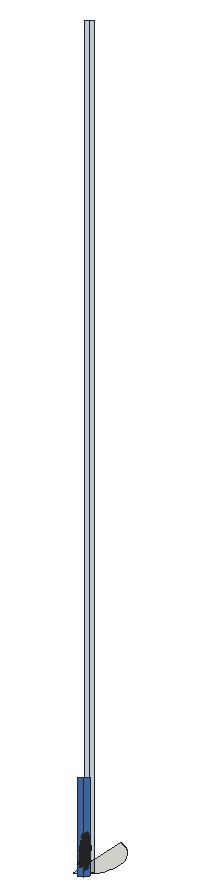
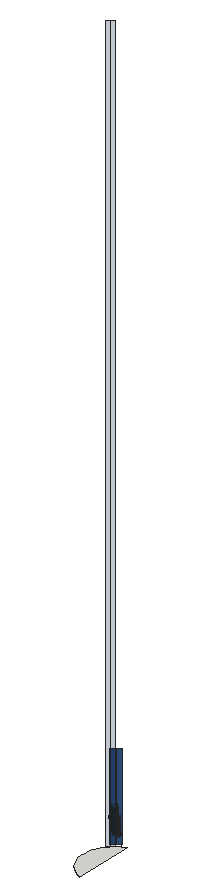
# SketchUp Ruby script. Lengths in inches.
U = 1.inch
M = Sketchup.active_model
def pt(a) = Geom::Point3d.new(a.map { |v| v * U })
def face(e, loops, mat)
  f = e.add_face(loops[0].map { |a| pt(a) })
  loops[1..].each { |l| e.add_face(l.map { |a| pt(a) }).erase! }
  f.material = f.back_material = mat if mat
  f
end
# faces: each face lists its corners as indices into pts; further lists are holes
def faces(e, pts, list, mat = nil) = list.each { |f| face(e, (f[0].is_a?(Array) ? f : [f]).map { |l| l.map { |i| pts[i] } }, mat) }
# xy, xz, yz: faces in a plane at the given z, y or x. An outline is a flat list of corners, or four numbers for a rectangle; further outlines are holes
def ring(l) = l.size == 4 ? [[l[0], l[1]], [l[2], l[1]], [l[2], l[3]], [l[0], l[3]]] : l.each_slice(2).to_a
def flat(e, list, mat, &to3) = list.each { |f| face(e, (f[0].is_a?(Array) ? f : [f]).map { |l| ring(l).map { |u, v| to3.(u, v) } }, mat) }
def xy(e, z, list, mat = nil) = flat(e, list, mat) { |x, y| [x, y, z] }
def xz(e, y, list, mat = nil) = flat(e, list, mat) { |x, z| [x, y, z] }
def yz(e, x, list, mat = nil) = flat(e, list, mat) { |y, z| [x, y, z] }
def lines(e, pts, list) = list.each { |a, b| e.add_line(pt(pts[a]), pt(pts[b])) }
# prism: a flat outline (further loops are holes) pulled along v
def prism(e, loops, v, mat = nil)
  f = face(e, loops, mat); d = Geom::Vector3d.new(v.map { |x| x * U })
  f.pushpull(f.normal.samedirection?(d) ? d.length : -d.length)
end
def box(e, o, s, mat = nil) = prism(e, [[o, [o[0] + s[0], o[1], o[2]], [o[0] + s[0], o[1] + s[1], o[2]], [o[0], o[1] + s[1], o[2]]]], [0, 0, s[2]], mat)
def at(x, y, z, deg = 0) = Geom::Transformation.translation(pt([x, y, z])) * Geom::Transformation.rotation(ORIGIN, Z_AXIS, deg.degrees)
def axes(o, x, y, z) = Geom::Transformation.new([*x, 0, *y, 0, *z, 0, *pt(o).to_a, 1])
def part(name) = M.definitions.add(name)
# library, detail: a bought-in or finely detailed component or shape, given as its bounding box
def library(name, o, s) = part(name).tap { |d| box(d.entities, o, s) }
def detail(e, o, s) = box(e.add_group.entities, o, s)
def put(e, d, t, mat = nil) = e.add_instance(d, t).tap { |i| i.material = mat if mat }
def group(e, t, mat = nil) = e.add_group.tap { |g| g.transformation = t; g.material = mat if mat }.entities
root = M.entities
M.materials.add("Glass_Basic_1").color = [0, 47, 91]
M.materials["Glass_Basic_1"].alpha = 0.25
M.materials.add("Glass_Mirror_01").color = [71, 118, 185]
M.materials.add("LightPink_Translucent").color = [144, 107, 117]
M.materials["LightPink_Translucent"].alpha = 0.75
c1 = part("blade")
p = [[2.15,0.21,22],[0,0.17,0],[0.09,0.45,0],[2.18,0.31,22],[2.29,0.31,22],[0.38,0.45,0],
  [2.48,0.24,33],[2.49,0.24,33],[2.48,0.22,33]]
faces(c1.entities,p,[[0,1,2,3],[4,5,2,3],[6,3,4,7],[8,0,3,6]])
c2 = part("seeds")
p = [[0.3,-0.1,1.38],[-0.01,-0.03,1.59],[-0.01,-0.03,0.03],[0.14,-0.07,-0.07],[0.29,-0.03,3],[0.15,0.01,3.11]]
faces(c2.entities,p,[[0,1,2,3],[1,0,4,5]],"LightPink_Translucent")
c3 = part("blade with seeds")
put(c3.entities,c1,at(0,0,0))
put(c3.entities,c2,axes([2.4,0.25,30.99],[1.5799,-0.05474,1.17369],[-0.12525,1.92788,0.29478],[-0.07173,-0.02425,1.56792]))
xy(root,-24,[[330.57,22.73,330.57,140.33,332.82,139.9,339.12,136.93,345.8,132.69,351.89,127.65,357.31,121.88,361.96,115.49,365.77,108.55,368.68,101.2,370.65,93.54,371.64,85.69,371.64,77.78,370.65,69.9375,368.68,62.28,365.77,54.92,361.96,47.99,357.31,41.59,351.89,35.83,345.8,30.78,339.12,26.55,331.97,23.18]])
p = [[351.1,23.49,-24],[351.1,23.49,150],[343.47,18.64,150],[343.47,18.64,-24],[358.07,29.25,-24],[358.07,29.25,150],
  [345.8,30.78,1482],[351.89,35.83,1482],[351.89,35.83,-24],[345.8,30.78,-24],[357.31,41.59,1482],[357.31,41.59,-24]]
faces(root,p,[[0,1,2,3],[4,5,1,0]],"Glass_Mirror_01")
faces(root,p,[[6,7,8,9],[7,10,11,8]],"Glass_Basic_1")
put(root,c3,axes([346.09,20.33,-5.23],[-0.00341,-0.09282,1.74944],[-0.28775,-0.26825,-0.27667],[0.04449,-0.16261,0.14031]))
put(root,c3,axes([344.7,21.5625,-7.89],[0.23773,-0.35053,-0.62353],[0.29532,0.31785,-0.16365],[0.09526,-0.08744,1.37633]))
put(root,c3,axes([345.71,20.84,-5.22],[0.25132,0.3182,0.48003],[-0.2669,0.27442,0.3958],[0.04636,-0.14929,0.9933]))
put(root,c3,axes([345.75,21.25,-7.92],[0.08291,0.40636,-0.30978],[-0.32928,0.11539,0.30978],[0.06638,0.04686,1.38974]))
put(root,c3,axes([346.36,22.58,-7.57],[0.44133,0,0],[0,0.52122,-0.51607],[0,0.11871,1.63711]))
put(root,c3,axes([344.9375,21.9,-7.28],[0.35635,-0.30962,-0.29095],[0.23697,0.43749,-0.50002],[0.08792,0.04443,1.59708]))
put(root,c3,axes([345.8,24.51,-7.28],[-0.22633,-0.01463,1.0506],[0.14947,-0.31064,0.58006],[0.08941,0.11036,0.8241]))
put(root,c3,axes([346,21.85,-4.9],[-0.30722,0.06665,0.35414],[-0.08112,-0.381,-0.4572],[0.08804,-0.10234,0.87481]))
put(root,c3,axes([345.11,20.78,-6.07],[-0.06572,0.16029,1.71376],[-0.27569,-0.33172,0.13857],[0.12437,-0.20675,0.73262]))
put(root,c3,axes([345.07,24.28,-4.91],[0.21031,-0.39918,-0.1216],[0.30457,0.22997,-0.67495],[0.10587,0.11278,1.02557]))
put(root,c3,axes([344.04,21.625,-8.36],[-0.3474,0.18671,1.28929],[-0.11057,-0.53572,0.50096],[0.21332,0.00891,1.46642]))
put(root,c3,axes([346.16,21.88,-4.91],[-0.32648,-0.25715,-0.1216],[0.18809,-0.3724,-0.67495],[0.09224,-0.12945,1.02557]))
put(root,c3,axes([345.32,24.08,-5.27],[0.34827,-0.11086,-0.51099],[0.06092,0.41983,-0.3958],[0.09354,0.12031,0.97773]))
put(root,c3,axes([345.64,20.8,-7.57],[0.22066,-0.46731,0],[0.36918,0.26061,-0.51607],[0.08408,0.05936,1.63711]))
put(root,c3,axes([346.01,20.59,-8.46],[-0.05283,-0.03674,1.76342],[-0.13569,-0.41045,-0.26939],[0.09154,-0.11138,0.30037]))
put(root,c3,axes([345.72,23.58,-4.9],[-0.20082,-0.29199,0.35414],[0.2293,-0.2764,-0.4572],[0.1165,0.04206,0.87481]))
put(root,c3,axes([345.84,21.08,-7.93],[0.33032,0.23318,-0.49651],[-0.19744,0.41812,0],[0.07523,0.05311,1.57504]))
put(root,c3,axes([345.9,23.84,-5.22],[-0.01777,0.35463,0.0643],[-0.26836,-0.00972,0.50621],[0.1028,0.03711,0.77189]))
put(root,c3,axes([345.82,24.4,-8.46],[0.02571,-0.06733,1.76342],[0.32373,-0.19829,-0.26939],[0.09815,0.10263,0.30037]))
put(root,c3,axes([345.92,23.73,-5.22],[-0.26024,0.30729,0.48003],[-0.22444,-0.32634,0.3958],[0.1221,0.05668,0.9933]))
put(root,c3,axes([345.99,21.58,-5.27],[-0.09067,-0.42583,-0.51099],[0.34336,-0.07449,-0.3958],[0.0984,-0.11438,0.97773]))
put(root,c3,axes([346.6,23.78,-6.02],[-0.06755,-0.39203,-0.03492],[0.31928,-0.09013,-0.15832],[0.06667,0.02485,0.52218]))
put(root,c3,axes([346.05,22.76,-4.9],[-0.29332,-0.1301,0.35414],[0.08555,-0.37955,-0.4572],[0.11809,-0.0348,0.87481]))
put(root,c3,axes([345.36,21.97,-7.89],[0.36714,0.07646,-0.62353],[-0.07747,0.47163,-0.16365],[0.10956,0.05715,1.37633]))
put(root,c3,axes([346.92,22.25,-7.6875],[-0.21881,-0.29821,-0.06488],[0.23965,-0.27324,-0.29416],[0.0679,-0.01924,0.97024]))
put(root,c3,axes([346.42,20.73,-7.18],[-0.11756,0.2374,1.1486],[-0.10105,-0.31895,0.84392],[0.09709,-0.07992,0.25299]))
put(root,c3,axes([346.28,21.79,-5.22],[0.2423,0.19613,0.0643],[-0.14107,0.2793,0.50621],[0.07768,-0.0903,0.77189]))
put(root,c3,axes([346.21,21.71,-5.22],[0.08753,0.42921,0.48003],[-0.34336,0.07449,0.3958],[0.1012,-0.10094,0.9933]))
put(root,c3,axes([345.28,22.98,-6.07],[-0.1311,-0.08035,1.71376],[0.27131,-0.33708,0.13857],[0.16909,0.15206,0.73262]))
put(root,c3,axes([346.96,21.77,-5.24],[-0.0461,-0.00354,1.77383],[-0.19143,-0.37951,-0.16761],[0.07688,-0.12478,0.31391]))
put(root,c3,axes([346.25,21.62,-5.42],[0.30722,-0.06665,-0.35414],[0.08112,0.381,0.4572],[0.08804,-0.10234,0.87481]))
put(root,c3,axes([346,21.75,-4.97],[0.18436,-0.36797,-0.71045],[0.32306,0.26151,0.08574],[0.11008,-0.13332,1.00501]))
put(root,c3,axes([346.3125,22.875,-5.22],[0.12963,0.31798,0.0643],[-0.23638,0.15564,0.50621],[0.1042,-0.03071,0.77189]))
put(root,c3,axes([346,23.73,-5.42],[0.20082,0.29199,-0.35414],[-0.2293,0.2764,0.4572],[0.1165,0.04206,0.87481]))
put(root,c3,axes([345.77,23.76,-4.91],[0.0189,-0.47427,-0.1216],[0.35781,0.01296,-0.67495],[0.13781,0.03295,1.02557]))
put(root,c3,axes([346.17,22.89,-4.91],[-0.17758,-0.42229,-0.1216],[0.31518,-0.20752,-0.67495],[0.13282,-0.05572,1.02557]))
put(root,c3,axes([346.29,22.76,-5.22],[-0.09971,0.42522,0.48003],[-0.32782,-0.1454,0.3958],[0.12892,-0.02555,0.9933]))
put(root,c3,axes([346.08,23.48,-5.23],[0.07571,-0.00789,1.74944],[0.20767,-0.36231,-0.27667],[0.13467,0.04783,0.14031]))
put(root,c3,axes([346.15,22.52,-5.27],[0.09562,-0.42421,-0.51099],[0.32782,0.1454,-0.3958],[0.13199,-0.0389,0.97773]))
put(root,c3,axes([346.98,22.79,-7.18],[-0.21807,0.07699,1.1486],[0.10265,-0.31819,0.84392],[0.11568,0.02177,0.25299]))
put(root,c3,axes([346.27,21.41,-7.36],[-0.12609,-0.01381,1.43002],[-0.12917,-0.37055,-0.30754],[0.1549,-0.10482,0.61141]))
put(root,c3,axes([346.36,22.72,-5.42],[0.29332,0.1301,-0.35414],[-0.08555,0.37955,0.4572],[0.11809,-0.0348,0.87481]))
put(root,c3,axes([345.79,23.54,-4.97],[0.35281,0.01123,-0.71045],[-0.0237,0.47284,0.08574],[0.14947,0.0499,1.00501]))
put(root,c3,axes([346.5,22.64,-7.97],[-0.22732,0.05597,1.41583],[-0.03618,-0.44548,0.08104],[0.15921,-0.06743,0.80566]))
put(root,c3,axes([346.75,22.35,-8.46],[-0.01845,-0.0708,1.76342],[0.12793,-0.41416,-0.26939],[0.12905,-0.00596,0.30037]))
put(root,c3,axes([346.875,24.14,-5.24],[-0.03191,-0.04083,1.77383],[0.06981,-0.43764,-0.16761],[0.12571,-0.02796,0.31391]))
put(root,c3,axes([345.56,22.25,-6.07],[-0.14639,0.01056,1.71376],[0.09712,-0.45778,0.13857],[0.20862,0.02831,0.73262]))
put(root,c3,axes([346.09,22.68,-4.97],[0.31014,-0.20596,-0.71045],[0.17284,0.42397,0.08574],[0.14985,-0.04816,1.00501]))
put(root,c3,axes([347.13,22.22,-5.23],[0.04898,-0.07104,1.74944],[-0.06269,-0.43574,-0.27667],[0.12289,-0.08262,0.14031]))
put(root,c3,axes([346.57,23.3,-7.36],[-0.085,-0.1147,1.43002],[0.1106,-0.37943,-0.30754],[0.17198,0.0514,0.61141]))
put(root,c3,axes([355.53,21.72,-6.45],[0.14639,-0.01056,1.71376],[-0.09712,0.45778,0.13857],[-0.20862,-0.02831,0.73262]))
put(root,c3,axes([355.59,22.52,-6.45],[0.12246,-0.09864,1.71376],[0.1031,0.45582,0.13857],[-0.19225,0.10302,0.73262]))
put(root,c3,axes([355.21,23.3,-7.73],[0.12266,0.03828,1.43002],[0.07906,0.39104,-0.30754],[-0.16661,0.0732,0.61141]))
put(root,c3,axes([356.29,22.05,-6.98],[0.10032,-0.06746,1.77064],[0.0346,0.47103,0.13857],[-0.2173,0.0625,0.63284]))
put(root,c3,axes([355.21,22.37,-5.61],[-0.05763,0.06055,1.74944],[0.0049,0.44239,-0.27667],[-0.13211,0.05753,0.14031]))
put(root,c3,axes([355.97,21.29,-5.34],[-0.35281,-0.01123,-0.71045],[0.0237,-0.47284,0.08574],[-0.14947,-0.0499,1.00501]))
put(root,c3,axes([355.68,21.41,-7.73],[0.06891,0.12984,1.43002],[-0.15879,0.35293,-0.30754],[-0.16304,-0.08436,0.61141]))
put(root,c3,axes([355.4,22.11,-5.8],[-0.29332,-0.1301,-0.35414],[0.08555,-0.37955,0.4572],[-0.11809,0.0348,0.87481]))
put(root,c3,axes([355.8,20.98,-6.45],[0.1311,0.08035,1.71376],[-0.27131,0.33708,0.13857],[-0.16909,-0.15206,0.73262]))
put(root,c3,axes([354.57,22.8125,-5.61],[0.04504,0.01251,1.77383],[0.13934,0.41205,-0.16761],[-0.0922,0.10815,0.31391]))
put(root,c3,axes([355.6,22.31,-5.64],[-0.09562,0.42421,-0.51099],[-0.32782,-0.1454,-0.3958],[-0.13199,0.0389,0.97773]))
put(root,c3,axes([355.85,21.39,-5.64],[-0.25628,0.30892,-0.51099],[-0.22444,-0.32634,-0.3958],[-0.13021,-0.047,0.97773]))
put(root,c3,axes([355.43,22.28,-8.83],[0.00895,0.0735,1.76342],[-0.18044,0.38382,-0.26939],[-0.12817,-0.01935,0.30037]))
put(root,c3,axes([355.49,20.52,-5.61],[0.02617,0.04654,1.77383],[-0.12614,0.41836,-0.16761],[-0.12775,0.00303,0.31391]))
put(root,c3,axes([354.95,24.12,-7.56],[0.14709,-0.21136,1.1486],[0.05804,0.3346,0.84392],[-0.1063,0.05991,0.25299]))
put(root,c3,axes([355.78,20.24,-5.61],[-0.07594,-0.00329,1.74944],[-0.24177,0.32918,-0.27667],[-0.129,-0.06726,0.14031]))
put(root,c3,axes([355.47,22.07,-5.59],[0.09971,-0.42522,0.48003],[0.32782,0.1454,0.3958],[-0.12892,0.02555,0.9933]))
put(root,c3,axes([355.58,21.94,-5.29],[0.17758,0.42229,-0.1216],[-0.31518,0.20752,-0.67495],[-0.13282,0.05572,1.02557]))
put(root,c3,axes([355.98,21.07,-5.29],[-0.0189,0.47427,-0.1216],[-0.35781,-0.01296,-0.67495],[-0.13781,-0.03295,1.02557]))
put(root,c3,axes([355.75,21.1,-5.8],[-0.20082,-0.29199,-0.35414],[0.2293,-0.2764,0.4572],[-0.1165,-0.04206,0.87481]))
put(root,c3,axes([355.44,21.95,-5.59],[-0.12963,-0.31798,0.0643],[0.23638,-0.15564,0.50621],[-0.1042,0.03071,0.77189]))
put(root,c3,axes([356.04,22.83,-6.45],[0.08815,-0.14329,1.71376],[0.22258,0.38678,0.13857],[-0.15267,0.17614,0.73262]))
put(root,c3,axes([355.51,23.21,-5.8],[-0.30722,0.06665,-0.35414],[-0.08112,-0.381,0.4572],[-0.08804,0.10234,0.87481]))
put(root,c3,axes([355.34,24.34,-8.83],[0.04734,0.04659,1.76342],[0.08027,0.4317,-0.26939],[-0.10492,0.09206,0.30037]))
put(root,c3,axes([355.27,21.8,-7.56],[0.22533,-0.03337,1.1486],[-0.14293,0.29403,0.84392],[-0.11135,-0.04411,0.25299]))
put(root,c3,axes([355.55,23.125,-5.59],[-0.08753,-0.42921,0.48003],[0.34336,-0.07449,0.3958],[-0.1012,0.10094,0.9933]))
put(root,c3,axes([355.72,20.99,-5.23],[0.29147,-0.34417,0.53763],[0.25138,0.3655,0.4433],[-0.13675,-0.06349,1.11249]))
put(root,c3,axes([355.48,23.04,-5.59],[-0.2423,-0.19613,0.0643],[0.14107,-0.2793,0.50621],[-0.07768,0.0903,0.77189]))
put(root,c3,axes([355.97,23.19,-6.45],[0.06572,-0.16029,1.71376],[0.27569,0.33172,0.13857],[-0.12437,0.20675,0.73262]))
put(root,c3,axes([355.71,22.07,-5.27],[0.29332,0.1301,0.35414],[-0.08555,0.37955,-0.4572],[-0.11809,0.0348,0.87481]))
put(root,c3,axes([355.76,23.25,-5.64],[0.09067,0.42583,-0.51099],[-0.34336,0.07449,-0.3958],[-0.0984,0.11438,0.97773]))
put(root,c3,axes([355.86,20.99,-5.59],[0.01777,-0.35463,0.0643],[0.26836,0.00972,0.50621],[-0.1028,-0.03711,0.77189]))
put(root,c3,axes([355.22,24.02,-5.61],[-0.00877,0.09229,1.74944],[0.24897,0.32105,-0.27667],[-0.06518,0.15182,0.14031]))
put(root,c3,axes([356.62,22.95,-8.26],[-0.36714,-0.07646,-0.62353],[0.07747,-0.47163,-0.16365],[-0.10956,-0.05715,1.37633]))
put(root,c3,axes([356.68,20.375,-4.89],[-0.23555,0.44708,-0.13619],[-0.34112,-0.25757,-0.75594],[-0.11858,-0.12631,1.14864]))
put(root,c3,axes([356.04,21.25,-5.27],[0.20082,0.29199,0.35414],[-0.2293,0.2764,-0.4572],[-0.1165,-0.04206,0.87481]))
put(root,c3,axes([356.58,20.74,-5.34],[-0.30095,-0.22541,-0.71045],[0.21388,-0.395,0.08574],[-0.10904,-0.13459,1.00501]))
put(root,c3,axes([356.4375,20.75,-5.64],[-0.34827,0.11086,-0.51099],[-0.06092,-0.41983,-0.3958],[-0.09354,-0.12031,0.97773]))
put(root,c3,axes([356.13,23.84,-8.3],[-0.33032,-0.23318,-0.49651],[0.19744,-0.41812,0],[-0.07523,-0.05311,1.57504]))
put(root,c3,axes([355.99,20.37,-8.83],[-0.03419,0.06144,1.76342],[-0.3455,0.13246,-0.26939],[-0.08346,-0.12049,0.30037]))
put(root,c3,axes([355.6,22.95,-5.29],[0.32648,0.25715,-0.1216],[-0.18809,0.3724,-0.67495],[-0.09224,0.12945,1.02557]))
put(root,c3,axes([356.33,24.12,-7.95],[-0.22066,0.46731,0],[-0.36918,-0.26061,-0.51607],[-0.08408,-0.05936,1.63711]))
put(root,c3,axes([355.06,24.0625,-4.68],[0.31145,0.12449,-0.06488],[-0.0958,0.38314,-0.29416],[-0.05094,0.05817,0.97024]))
put(root,c3,axes([355.76,22.98,-5.27],[0.30722,-0.06665,0.35414],[0.08112,0.381,-0.4572],[-0.08804,0.10234,0.87481]))
put(root,c3,axes([355.93,24.8,-7.73],[0.11138,-0.07357,1.43002],[0.27499,0.22183,-0.30754],[-0.08185,0.19194,0.61141]))
put(root,c3,axes([355.77,20.6,-8.19],[-0.10181,0.3808,-0.03893],[-0.31336,-0.11714,-0.17649],[-0.04758,-0.06228,0.58215]))
put(root,c3,axes([356.59,19.31,-5.61],[-0.00658,0.0559,1.77383],[-0.32474,0.20287,-0.16761],[-0.09556,-0.1037,0.31391]))
put(root,c3,axes([356.24,20.12,-7.73],[-0.02137,0.15256,1.43002],[-0.31245,0.12771,-0.30754],[-0.07303,-0.19719,0.61141]))
put(root,c3,axes([356.34,20.52,-6.45],[0.08068,0.14973,1.71376],[-0.3728,0.12606,0.13857],[-0.08426,-0.23506,0.73262]))
put(root,c3,axes([357.03,23.02,-7.66],[-0.35635,0.30962,-0.29095],[-0.23697,-0.43749,-0.50002],[-0.08792,-0.04443,1.59708]))
put(root,c3,axes([356.05,23.99,-5.59],[-0.25132,-0.3182,0.48003],[0.2669,-0.27442,0.3958],[-0.04636,0.14929,0.9933]))
put(root,c3,axes([356.47,20.4375,-5.8],[-0.05451,-0.37564,-0.35414],[0.31161,-0.09919,0.4572],[-0.0837,-0.10765,0.87481]))
put(root,c3,axes([355.61,22.34,-7.95],[-0.44133,0,0],[0,-0.52122,-0.51607],[0,-0.11871,1.63711]))
put(root,c3,axes([356.23,23.66,-8.29],[-0.08291,-0.40636,-0.30978],[0.32928,-0.11539,0.30978],[-0.06638,-0.04686,1.38974]))
put(root,c3,axes([355.95,23.96,-5.59],[-0.29004,-0.02173,0.0643],[0.00795,-0.32812,0.50621],[-0.03035,0.12569,0.77189]))
put(root,c3,axes([356.05,24.09,-5.8],[-0.23881,0.24554,-0.35414],[-0.22606,-0.28036,0.4572],[-0.0344,0.14245,0.87481]))
put(root,c3,axes([357.27,23.35,-8.26],[-0.23773,0.35053,-0.62353],[-0.29532,-0.31785,-0.16365],[-0.09526,0.08744,1.37633]))
put(root,c3,axes([356.66,20.74,-5.27],[0.05451,0.37564,0.35414],[-0.31161,0.09919,-0.4572],[-0.0837,-0.10765,0.87481]))
put(root,c3,axes([355.19,24.96,-5.61],[0.04004,-0.02816,1.77383],[0.33095,0.18728,-0.16761],[-0.00778,0.15594,0.31391]))
put(root,c3,axes([355.95,22.2,-7.99],[-0.32829,0.39208,0.30756],[-0.32849,-0.38796,-0.36492],[-0.01146,-0.11134,1.64885]))
put(root,c3,axes([357.3,23.29,-7],[0.305,0.18805,1.51261],[-0.29879,0.40513,0.59816],[-0.13384,-0.24012,1.26806]))
put(root,c3,axes([356.13,19.875,-7.56],[0.18411,0.16231,1.1486],[-0.26813,0.09757,0.84392],[-0.05737,-0.12474,0.25299]))
put(root,c3,axes([357.43,23.16,-7.86],[-0.34464,-0.37536,-0.25192],[0.29,-0.42149,0.5513],[-0.0928,0.04391,1.68216]))
put(root,c3,axes([356.81,22.8,-8.11],[-0.21202,-0.39143,-0.44739],[0.32115,-0.27564,0.21531],[-0.06861,-0.04843,1.43643]))
put(root,c3,axes([356.21,23.83,-4.98],[-0.00918,0.43138,-0.7886],[-0.38672,-0.02897,0.09517],[-0.04081,0.18275,1.11556]))
put(root,c3,axes([356.2,25.04,-7.56],[-0.00913,-0.2773,1.1486],[0.22824,0.19778,0.84392],[-0.04489,0.13217,0.25299]))
put(root,c3,axes([356.52,20.3,-5.23],[0.39316,-0.11987,0.53763],[0.06823,0.47021,0.4433],[-0.09247,-0.13858,1.11249]))
put(root,c3,axes([357.26,23.08,-8.11],[-0.38326,0.02879,-0.44739],[-0.03466,-0.47788,0.21531],[-0.06861,0.04843,1.43643]))
put(root,c3,axes([356.61,20.4,-5.59],[0.16041,-0.29625,0.0643],[0.22843,0.17248,0.50621],[-0.07385,-0.09498,0.77189]))
put(root,c3,axes([356.52,23.875,-7.84],[0.33032,0.23318,0.49651],[-0.19744,0.41812,0],[-0.07523,-0.05311,1.57504]))
put(root,c3,axes([356.08,24.4375,-6.96],[0.00775,-0.24075,1.54345],[0.34877,0.12716,0.21329],[-0.03022,0.25658,0.72882]))
put(root,c3,axes([356.84,23.02,-7.88],[0.09355,-0.55261,-0.23429],[0.44354,0.09633,0.51271],[-0.0775,-0.07631,1.5644]))
put(root,c3,axes([357,23.15,-7.71],[-0.06809,0.4162,0.1448],[-0.33266,-0.07225,-0.41347],[-0.06054,-0.04274,1.26744]))
put(root,c3,axes([356.96,19.52,-5.61],[-0.05398,-0.06539,1.74944],[-0.36026,0.04145,-0.27667],[-0.0575,-0.15639,0.14031]))
put(root,c3,axes([357.66,24.31,-8.3],[-0.33032,0.23318,-0.49651],[-0.19744,-0.41812,0],[-0.07523,0.05311,1.57504]))
put(root,c3,axes([355.7,21.99,-8.3],[0,-0.46636,-0.49651],[0.39487,0,0],[0,-0.10622,1.57504]))
put(root,c3,axes([355.875,22.42,-7.84],[0,0.46636,0.49651],[-0.39487,0,0],[0,-0.10622,1.57504]))
put(root,c3,axes([357.68,24.19,-8.13],[-0.21791,-0.46895,-0.05142],[0.36918,-0.26061,0.51607],[-0.09097,0.04465,1.6363]))
put(root,c3,axes([356.28,23.97,-5.32],[0.25266,0.31335,-0.5672],[-0.2669,0.27442,-0.43934],[-0.03844,0.15921,1.08528]))
put(root,c3,axes([357.58,24.125,-8.29],[-0.32928,-0.11539,-0.30978],[0.08291,-0.40636,0.30978],[-0.06638,0.04686,1.38974]))
put(root,c3,axes([356.17,23.74,-5.27],[0.23881,-0.24554,0.35414],[0.22606,0.28036,-0.4572],[-0.0344,0.14245,0.87481]))
put(root,c3,axes([356.74,22.53,-7.66],[-0.39748,-0.22252,-0.29095],[0.19139,-0.46966,-0.50002],[-0.01249,-0.11531,1.59708]))
put(root,c3,axes([357.77,22.39,-7.48],[-0.00964,-0.43909,1.41272],[0.43635,0.11382,0.59816],[-0.1032,0.24027,1.3335]))
put(root,c3,axes([356.02,23.81,-4.92],[0.3879,0.02311,-0.13498],[-0.0106,0.43749,-0.74919],[-0.02694,0.1685,1.13838]))
put(root,c3,axes([356.01,24.44,-7.5],[0.32063,-0.08258,0.06507],[0.07371,0.33271,-0.86304],[-0.02033,0.16842,0.7736]))
put(root,c3,axes([357.53,22.95,-7.66],[0.04113,0.53214,-0.29095],[-0.42835,0.03218,-0.50002],[-0.07543,0.07088,1.59708]))
put(root,c3,axes([356.56,22.05,-8.22],[-0.14494,-0.47823,-0.69835],[0.41752,-0.17223,-0.18329],[-0.01602,-0.16194,1.54149]))
put(root,c3,axes([357.51,20.53,-5.29],[-0.34538,0.21713,-0.1216],[-0.16972,-0.38536,-0.67495],[-0.04557,-0.16239,1.02557]))
put(root,c3,axes([357.21,20.55,-5.64],[-0.34695,-0.11691,-0.51099],[0.11892,-0.40083,-0.3958],[-0.03181,-0.16138,0.97773]))
put(root,c3,axes([356.57,23.52,-6.45],[-0.00864,-0.17899,1.71376],[0.37441,0.11874,0.13857],[-0.02316,0.25508,0.73262]))
put(root,c3,axes([355.875,22,-8.29],[0.24637,-0.29097,-0.30978],[0.24637,0.29097,0.30978],[0,-0.09372,1.38974]))
put(root,c3,axes([356.99,20.12,-8.19],[-0.2439,0.26754,-0.03893],[-0.22348,-0.29302,-0.17649],[-0.01573,-0.08303,0.58215]))
put(root,c3,axes([356.89,22.75,-7.96],[0.44609,0.09826,0.45755],[-0.09078,0.55493,0.17955],[-0.06519,-0.05359,1.58856]))
put(root,c3,axes([356.77,22.65,-7.6],[-0.17124,0.42022,0.44739],[-0.35581,-0.20224,-0.21531],[0,-0.09687,1.43643]))
put(root,c3,axes([357.34,20.63,-5.34],[-0.16845,-0.3792,-0.71045],[0.34676,-0.21133,0.08574],[-0.03939,-0.18322,1.00501]))
put(root,c3,axes([356.65,23.64,-7.85],[0.37926,-0.12378,0.17642],[0.09365,0.46065,0.35086],[-0.03382,-0.06712,1.60407]))
put(root,c3,axes([357.14,23.71,-8.125],[-0.35581,-0.20937,0],[0.17124,-0.43505,0],[0,0,1.62707]))
put(root,c3,axes([357.4,20.68,-5.27],[-0.1064,0.35863,0.35414],[-0.31043,-0.1046,-0.4572],[-0.02846,-0.14439,0.87481]))
put(root,c3,axes([357.96,24.24,-7.95],[0.22066,0.46731,0],[-0.36918,0.26061,-0.51607],[-0.08408,0.05936,1.63711]))
put(root,c3,axes([356.84,24.4375,-5.26],[-0.34777,-0.12192,0.53283],[0.11892,-0.40083,0.43934],[0.0209,0.15763,1.10256]))
put(root,c3,axes([356.74,24.47,-5.59],[-0.26007,0.1585,0.0643],[-0.12729,-0.28902,0.50621],[0.02512,0.1274,0.77189]))
put(root,c3,axes([357.78,23.67,-7.85],[0.10196,-0.46348,0.17642],[0.3731,0.13116,0.35086],[-0.06445,0.00226,1.60407]))
put(root,c3,axes([357.6,23.05,-7.71],[0.26075,0.2802,0.1448],[-0.2175,0.31612,-0.41347],[-0.06054,0.04274,1.26744]))
put(root,c3,axes([357.51,22.71,-8.02],[-0.32829,-0.4014,-0.06131],[0.32849,-0.40164,0],[-0.01146,-0.01402,1.75571]))
put(root,c3,axes([357.6,22.85,-7.6],[0.38326,-0.02879,0.44739],[0.03466,0.47788,-0.21531],[-0.06861,0.04843,1.43643]))
put(root,c3,axes([357.69,23.94,-7.99],[0.44186,0.15158,0.30756],[-0.11054,0.54181,-0.36492],[-0.07313,0.06781,1.64885]))
put(root,c3,axes([357.05,19.79,-8.83],[-0.0592,0.0168,1.76342],[-0.32738,-0.18913,-0.26939],[0.00549,-0.15776,0.30037]))
put(root,c3,axes([357.88,23.91,-7.84],[0.33032,-0.23318,0.49651],[0.19744,0.41812,0],[-0.07523,0.05311,1.57504]))
put(root,c3,axes([357.37,20.31,-5.8],[0.1064,-0.35863,-0.35414],[0.31043,0.1046,0.4572],[-0.02846,-0.14439,0.87481]))
put(root,c3,axes([356.85,22.24,-7.96],[0.15345,0.52148,0.45755],[-0.43845,0.18134,0.17955],[0.00536,-0.09582,1.58856]))
put(root,c3,axes([356.78,22.18,-8.11],[0.17124,-0.42022,-0.44739],[0.35581,0.20224,0.21531],[0,-0.09687,1.43643]))
put(root,c3,axes([357.22,23.53,-8.12],[-0.11516,-0.40207,0],[0.32884,-0.1408,0],[0,0,1.54371]))
put(root,c3,axes([356.8,24.38,-8.83],[0.05712,-0.02538,1.76342],[0.34359,0.13968,-0.26939],[0.01005,0.15742,0.30037]))
put(root,c3,axes([356.875,24.52,-5.8],[-0.1064,0.35863,-0.35414],[-0.31043,-0.1046,0.4572],[0.02846,0.14439,0.87481]))
put(root,c3,axes([357.68,22.74,-8.11],[-0.17124,0.42022,-0.44739],[-0.35581,-0.20224,0.21531],[0,0.09687,1.43643]))
put(root,c3,axes([357.5,20.36,-5.59],[0.26007,-0.1585,0.0643],[0.12729,0.28902,0.50621],[-0.02512,-0.1274,0.77189]))
put(root,c3,axes([356.66,25.16,-5.61],[0.04474,0.0751,1.74944],[0.36104,0.0295,-0.27667],[0.03631,0.16562,0.14031]))
put(root,c3,axes([358.36,22.48,-7.85],[-0.2773,-0.3397,0.17642],[0.27945,-0.32949,0.35086],[-0.03063,0.06937,1.60407]))
put(root,c3,axes([357.4,22.29,-8.12],[0,-0.53961,0],[0.44133,0,0],[0,0,1.79456]))
put(root,c3,axes([357.41,20.39,-5.59],[0.34777,0.12192,0.48003],[-0.11892,0.40083,0.3958],[-0.0209,-0.15763,0.9933]))
put(root,c3,axes([356.99,22.39,-7.89],[0.39767,0.22603,0.24065],[-0.19139,0.46966,0.50002],[0,-0.10827,1.60543]))
put(root,c3,axes([357.625,22.5,-8.03],[0,0.53934,-0.05637],[-0.44133,0,0],[0,0.01695,1.79368]))
put(root,c3,axes([356.86,22.07,-7.6],[-0.38326,0.02879,0.44739],[-0.03466,-0.47788,-0.21531],[0.06861,-0.04843,1.43643]))
put(root,c3,axes([356.84,24.14,-5.27],[0.1064,-0.35863,0.35414],[0.31043,0.1046,-0.4572],[0.02846,0.14439,0.87481]))
put(root,c3,axes([356.68,21.25,-7.85],[-0.10196,0.46348,0.17642],[-0.3731,-0.13116,0.35086],[0.06445,-0.00226,1.60407]))
put(root,c3,axes([357.41,23.55,-8.03],[0.15345,0.53576,-0.06012],[-0.43845,0.18773,0],[0.00536,0.01871,1.72173]))
put(root,c3,axes([356.5,20.68,-7.95],[-0.22066,-0.46731,0],[0.36918,-0.26061,-0.51607],[0.08408,-0.05936,1.63711]))
put(root,c3,axes([356.91,24.2,-5.34],[0.16845,0.3792,-0.71045],[-0.34676,0.21133,0.08574],[0.03939,0.18322,1.00501]))
put(root,c3,axes([358.68,22.84,-8.12],[-0.44111,-0.00373,-0.04976],[0,-0.52122,0.49943],[-0.01386,0.11865,1.58352]))
put(root,c3,axes([357.8125,21.28,-7.85],[-0.37926,0.12378,0.17642],[-0.09365,-0.46065,0.35086],[0.03382,0.06712,1.60407]))
put(root,c3,axes([357.43,19.55,-7.56],[0.04528,0.27194,1.1486],[-0.25117,-0.15062,0.84392],[0.02703,-0.13924,0.25299]))
put(root,c3,axes([357.26,25.42,-4.68],[0.2439,-0.26754,-0.06488],[0.22348,0.29302,-0.29416],[0.01573,0.08303,0.97024]))
put(root,c3,axes([357.19,21.95,-7.96],[-0.29264,0.42323,0.45755],[-0.34767,-0.3736,0.17955],[0.07055,-0.04224,1.58856]))
put(root,c3,axes([357.69,22.62,-8.11],[0.24637,0.30123,0],[-0.24637,0.30123,0],[0,0,1.69266]))
put(root,c3,axes([357.6875,22.26,-7.6],[0.17124,-0.42022,0.44739],[0.35581,0.20224,-0.21531],[0,0.09687,1.43643]))
put(root,c3,axes([357.54,23.72,-8.12],[0.35581,0.20937,0],[-0.17124,0.43505,0],[0,0,1.74954]))
put(root,c3,axes([357.03,24.28,-5.64],[0.34695,0.11691,-0.51099],[-0.11892,0.40083,-0.3958],[0.03181,0.16138,0.97773]))
put(root,c3,axes([356.74,24.3,-5.29],[0.34538,-0.21713,-0.1216],[0.16972,0.38536,-0.67495],[0.04557,0.16239,1.02557]))
put(root,c3,axes([357.57,22.16,-7.94],[-0.44609,-0.09826,0.49198],[0.09078,-0.55493,0.19306],[0.06519,0.05359,1.70813]))
put(root,c3,axes([358.5,19.99,-5.61],[-0.03584,0.03562,1.77383],[-0.35118,-0.12018,-0.16761],[-0.01271,-0.15545,0.31391]))
put(root,c3,axes([358.23,21.02,-5.29],[-0.3879,-0.02311,-0.1216],[0.0106,-0.43749,-0.67495],[0.02694,-0.1685,1.02557]))
put(root,c3,axes([358.59,22.92,-8.29],[-0.24637,0.29097,-0.30978],[-0.24637,-0.29097,0.30978],[0,0.09372,1.38974]))
put(root,c3,axes([357.88,22.87,-8.23],[0.12941,0.42699,-0.69212],[-0.37279,0.15378,-0.18165],[0.0143,0.14459,1.52773]))
put(root,c3,axes([357.7,22.41,-8.12],[0.39487,0,0],[0,0.48281,0],[0,0,1.78407]))
put(root,c3,axes([358.07,21.09,-5.27],[-0.23881,0.24554,0.35414],[-0.22606,-0.28036,-0.4572],[0.0344,-0.14245,0.87481]))
put(root,c3,axes([357.32,21.875,-7.6],[-0.21202,-0.39143,0.44739],[0.32115,-0.27564,-0.21531],[0.06861,0.04843,1.43643]))
put(root,c3,axes([356.94,21.97,-7.66],[-0.04113,-0.53214,-0.29095],[0.42835,-0.03218,-0.50002],[0.07543,-0.07088,1.59708]))
put(root,c3,axes([357.84,22.36,-7.71],[0.32884,-0.136,0.1448],[0.11516,0.38837,-0.41347],[0,0.08547,1.26744]))
put(root,c3,axes([357.96,20.86,-5.64],[-0.25266,-0.31335,-0.51099],[0.2669,-0.27442,-0.3958],[0.03844,-0.15921,0.97773]))
put(root,c3,axes([357.72,22.39,-7.66],[0.39748,0.22252,-0.29095],[-0.19139,0.46966,-0.50002],[0.01249,0.11531,1.59708]))
put(root,c3,axes([356.88,20.79,-8.29],[0.32928,0.11539,-0.30978],[-0.08291,0.40636,0.30978],[0.06638,-0.04686,1.38974]))
put(root,c3,axes([357.79,20.3,-7.73],[-0.10032,0.0944,1.43002],[-0.30046,-0.16522,-0.30754],[0.05569,-0.20547,0.61141]))
put(root,c3,axes([358.59,22.5,-7.84],[0,-0.46636,0.49651],[0.39487,0,0],[0,0.10622,1.57504]))
put(root,c3,axes([358.76,22.93,-8.3],[0,0.46636,-0.49651],[-0.39487,0,0],[0,0.10622,1.57504]))
